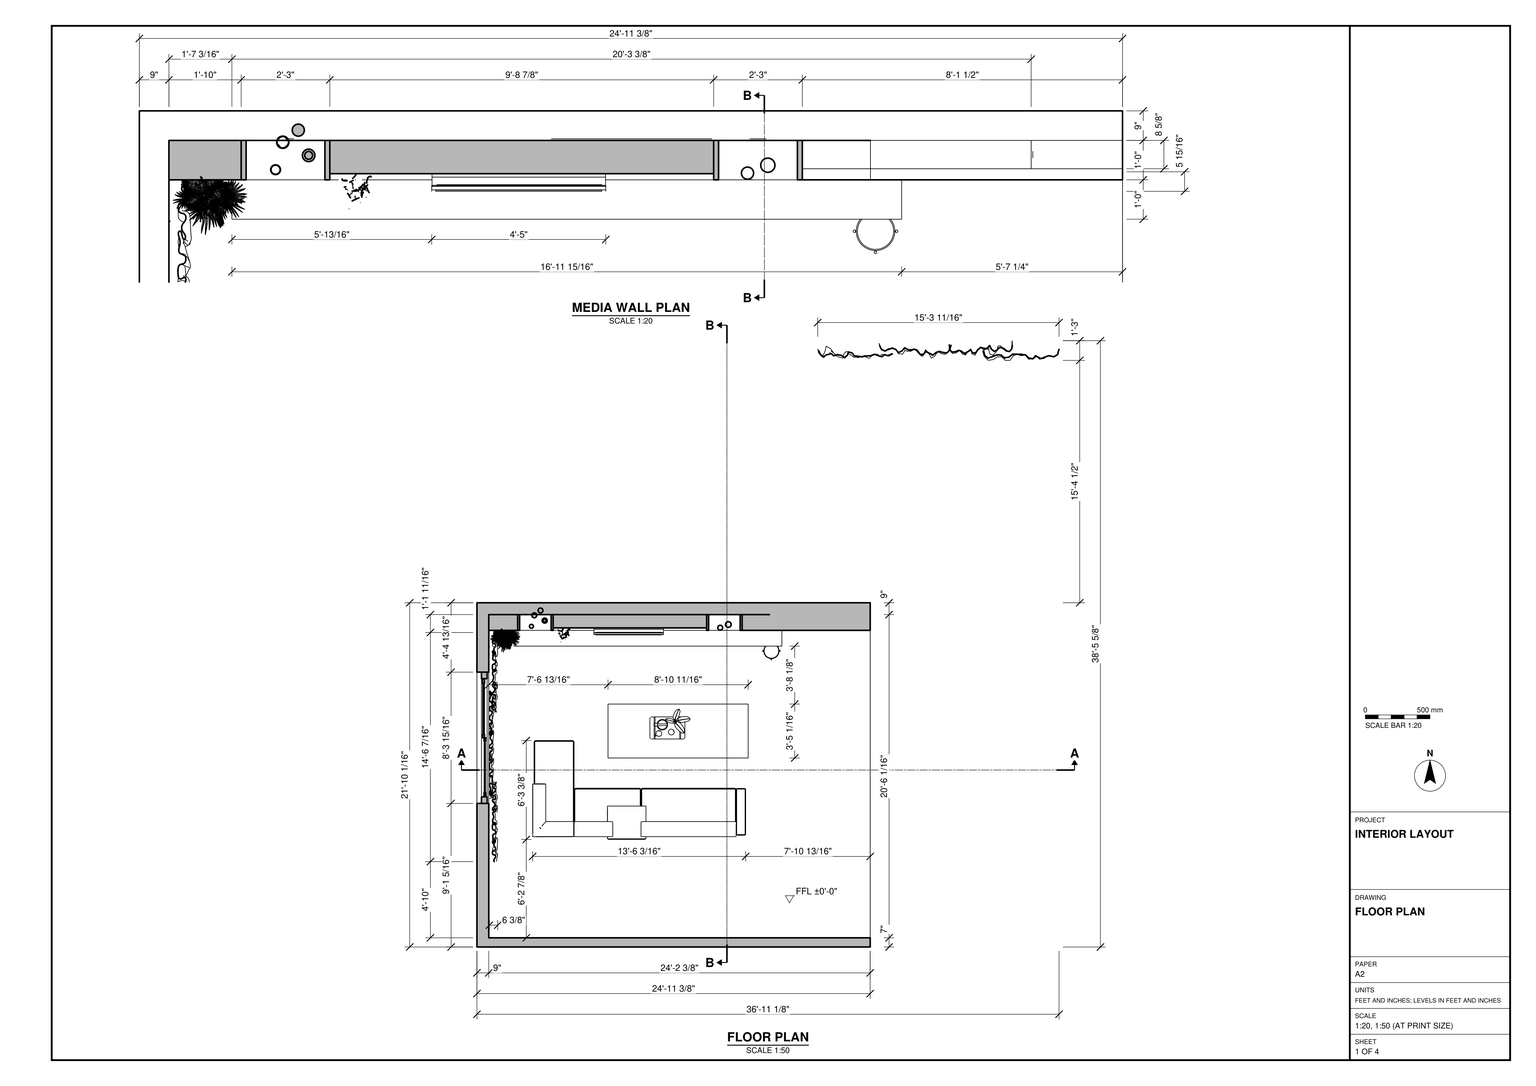
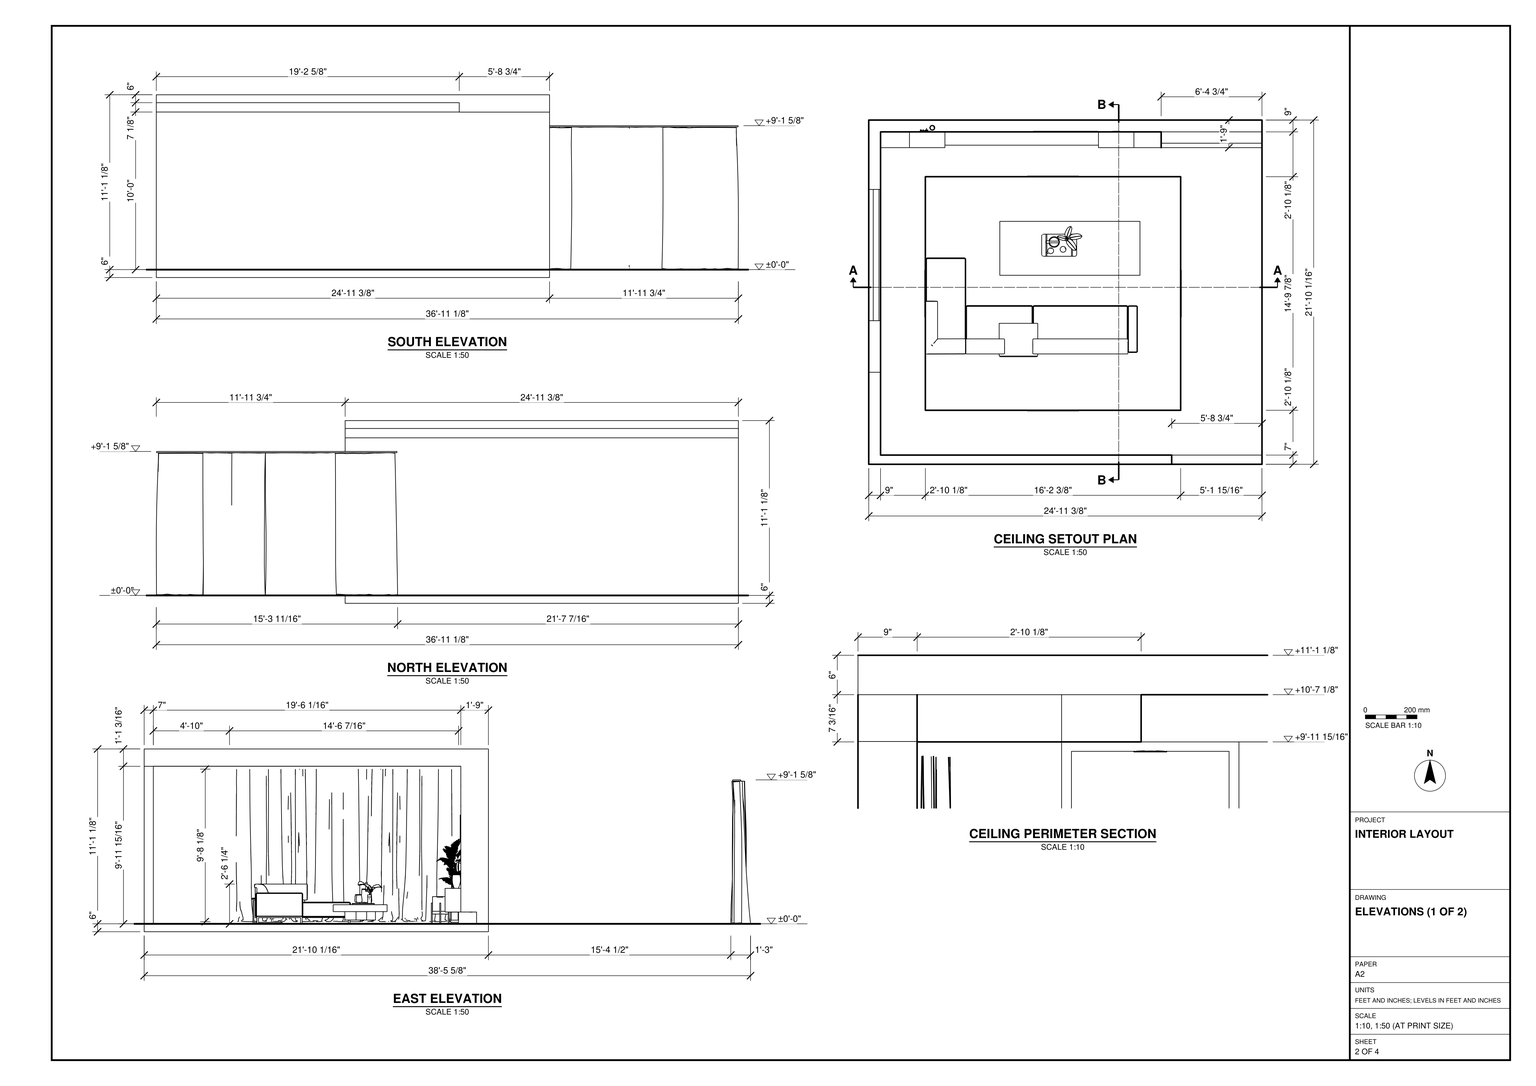
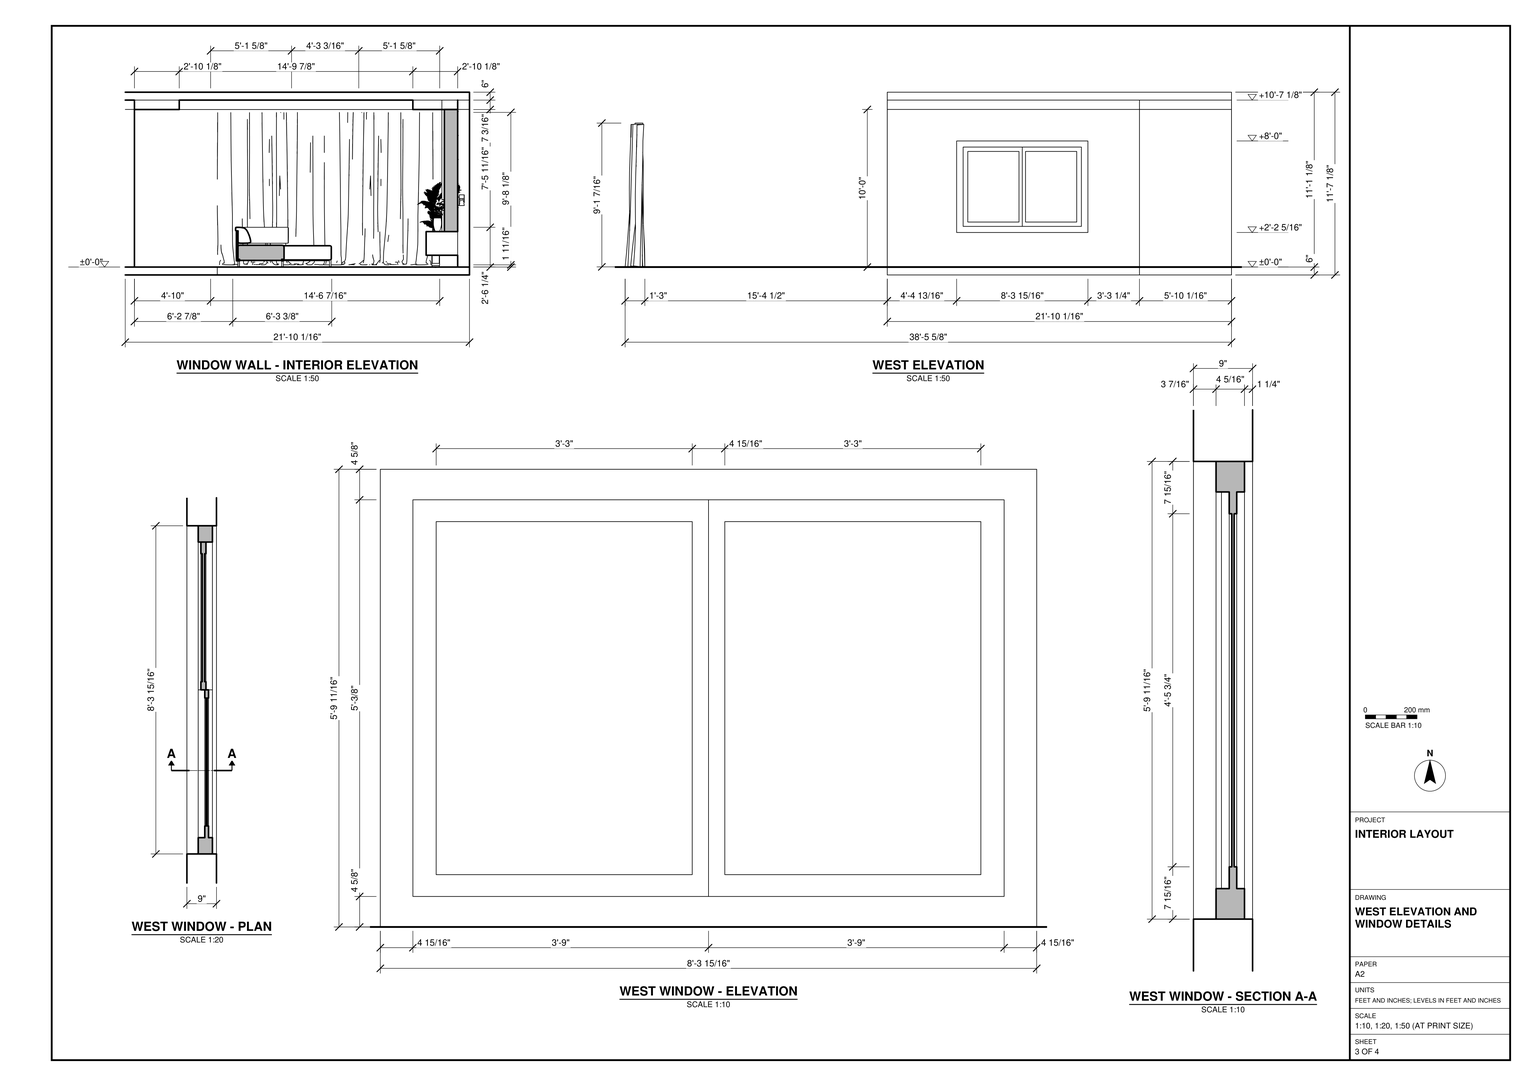
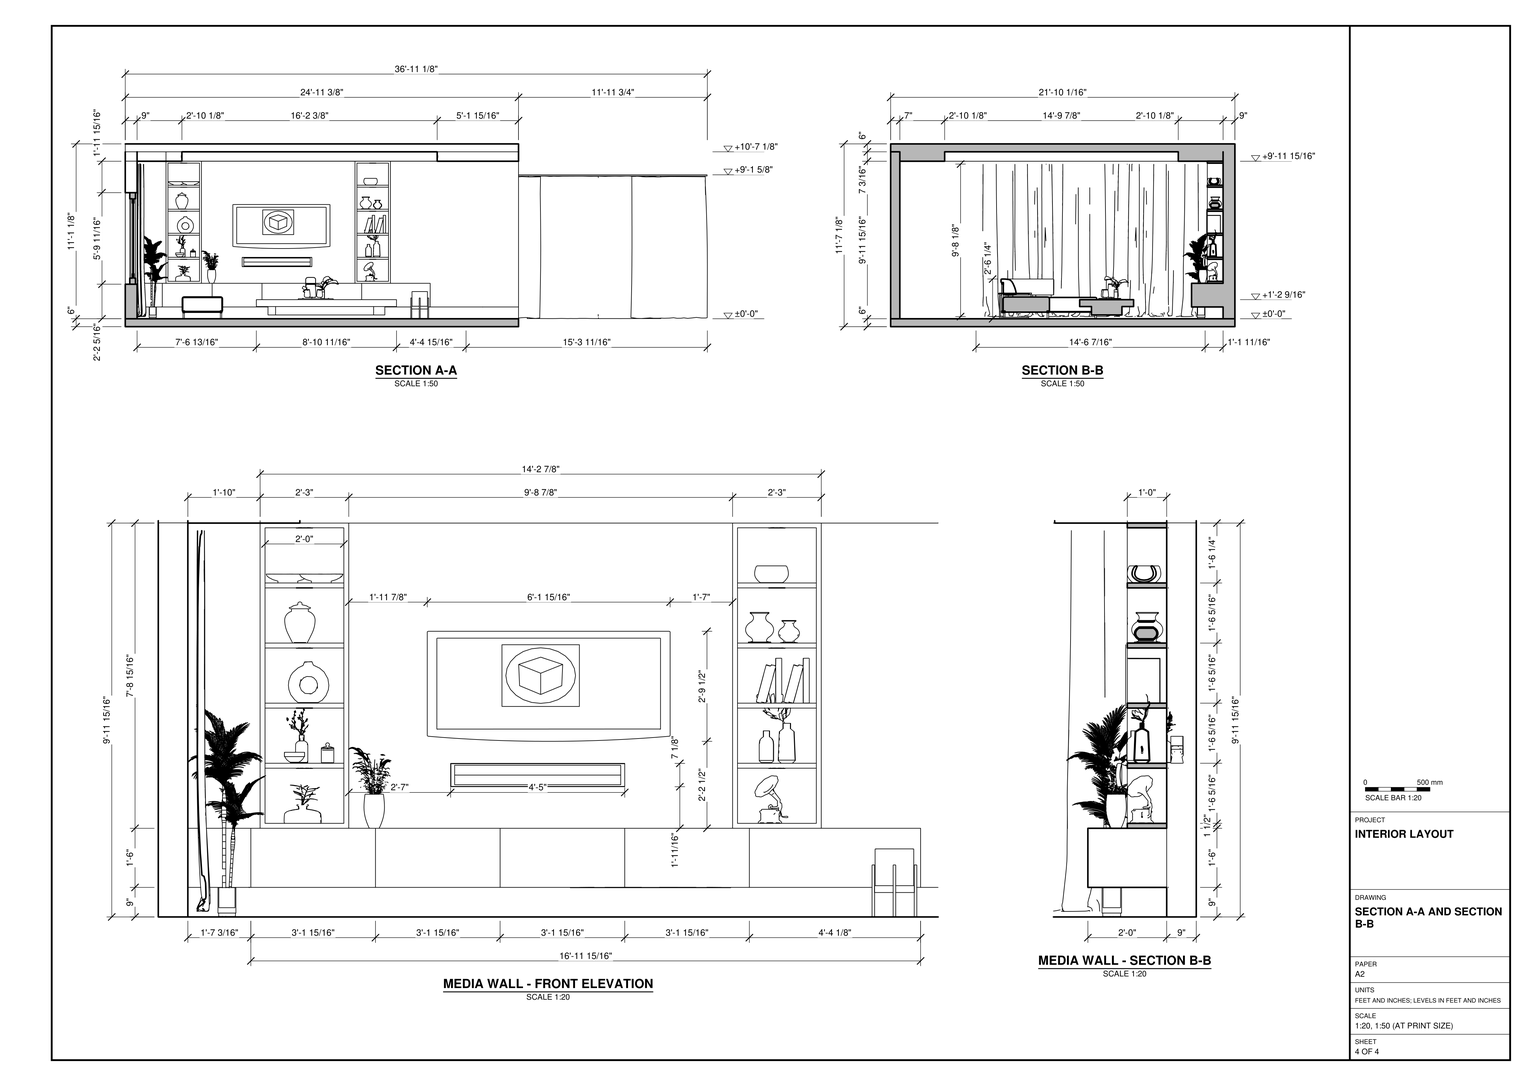
Build the living-room interior in SketchUp from task_files/diagram_01.pdf. Work in feet and inches, with the finished floor at ±0'-0". The complete model measures 36'-11 1/8" along X, 38'-5 5/8" along Y and 11'-7 1/8" along Z. These are not the room dimensions: the room shell measures 24'-11 3/8" across the media wall by 21'-10 1/16" along the window wall. Include the separate curtain run beyond the room where the floor plan and elevations show it.

Build the floor slab, the north and west walls at 9" thick and the south wall at 7" thick. Leave the east side open as drawn. Use the ceiling setout and perimeter section to form the lowered border around the recessed ceiling. Set the paired window into the west wall, with its frame, sill height and glazing taken from the window details, and place the interior curtains along that wall.

Use the enlarged media wall plan to set out the built-in bays, screen and projecting low unit on the north wall. Place the sectional sofa facing the screen, with its short return on the window side and the rectangular coffee table between the sofa and the media wall. Decor and loose items may be any suitable library components placed as shown. Keep shell elements and each furniture or joinery piece in separate groups or components, using components for repeated parts. Save one SketchUp model as output_files/living_room_with_its_media_wall_and_sectional_sofa.skp.

# SketchUp Ruby script. Lengths in inches.
U = 1.inch
M = Sketchup.active_model
def pt(a) = Geom::Point3d.new(a.map { |v| v * U })
def face(e, loops, mat)
  f = e.add_face(loops[0].map { |a| pt(a) })
  loops[1..].each { |l| e.add_face(l.map { |a| pt(a) }).erase! }
  f.material = f.back_material = mat if mat
  f
end
# faces: each face lists its corners as indices into pts; further lists are holes
def faces(e, pts, list, mat = nil) = list.each { |f| face(e, (f[0].is_a?(Array) ? f : [f]).map { |l| l.map { |i| pts[i] } }, mat) }
# xy, xz, yz: faces in a plane at the given z, y or x. An outline is a flat list of corners, or four numbers for a rectangle; further outlines are holes
def ring(l) = l.size == 4 ? [[l[0], l[1]], [l[2], l[1]], [l[2], l[3]], [l[0], l[3]]] : l.each_slice(2).to_a
def flat(e, list, mat, &to3) = list.each { |f| face(e, (f[0].is_a?(Array) ? f : [f]).map { |l| ring(l).map { |u, v| to3.(u, v) } }, mat) }
def xy(e, z, list, mat = nil) = flat(e, list, mat) { |x, y| [x, y, z] }
def xz(e, y, list, mat = nil) = flat(e, list, mat) { |x, z| [x, y, z] }
def yz(e, x, list, mat = nil) = flat(e, list, mat) { |y, z| [x, y, z] }
def lines(e, pts, list) = list.each { |a, b| e.add_line(pt(pts[a]), pt(pts[b])) }
# prism: a flat outline (further loops are holes) pulled along v
def prism(e, loops, v, mat = nil)
  f = face(e, loops, mat); d = Geom::Vector3d.new(v.map { |x| x * U })
  f.pushpull(f.normal.samedirection?(d) ? d.length : -d.length)
end
def box(e, o, s, mat = nil) = prism(e, [[o, [o[0] + s[0], o[1], o[2]], [o[0] + s[0], o[1] + s[1], o[2]], [o[0], o[1] + s[1], o[2]]]], [0, 0, s[2]], mat)
def at(x, y, z, deg = 0) = Geom::Transformation.translation(pt([x, y, z])) * Geom::Transformation.rotation(ORIGIN, Z_AXIS, deg.degrees)
def axes(o, x, y, z) = Geom::Transformation.new([*x, 0, *y, 0, *z, 0, *pt(o).to_a, 1])
def part(name) = M.definitions.add(name)
# library, detail: a bought-in or finely detailed component or shape, given as its bounding box
def library(name, o, s) = part(name).tap { |d| box(d.entities, o, s) }
def detail(e, o, s) = box(e.add_group.entities, o, s)
def put(e, d, t, mat = nil) = e.add_instance(d, t).tap { |i| i.material = mat if mat }
def group(e, t, mat = nil) = e.add_group.tap { |g| g.transformation = t; g.material = mat if mat }.entities
root = M.entities
M.materials.add("Generic").color = [37, 72, 93]
M.materials.add("Generic\#1").color = [217, 232, 252]
M.materials.add("Generic\#2").color = [244, 244, 245]
M.materials.add("Generic\#3").color = [100, 110, 121]
M.materials.add("[Translucent Glass Gray]").color = [128, 128, 128]
M.materials["[Translucent Glass Gray]"].alpha = 0.5
M.materials.add("[Translucent_Glass_Safety]").color = [204, 235, 244]
M.materials["[Translucent_Glass_Safety]"].alpha = 0.5
M.materials.add("[Translucent_Glass_Sky_Reflection]").color = [125, 138, 183]
M.materials["[Translucent_Glass_Sky_Reflection]"].alpha = 0.52
c1 = part("Sliding window")
xy(c1.entities,0,[[0,0,4.33,55.51]])
xy(c1.entities,2.76,[[0,2.76,2,27.76],[3.15,2.76,4.33,27.76],[0,27.76,0.82,52.76],[0.82,27.76,2.36,52.76],[2.36,27.76,4.33,52.76]])
xy(c1.entities,4.72,[[2,4.72,2.4,26.38],[2.76,4.72,3.15,26.38],[0.82,29.13,1.22,50.79],[1.97,29.13,2.36,50.79]])
xy(c1.entities,36.61,[[2,4.72,2.4,26.38],[2.76,4.72,3.15,26.38],[0.82,29.13,1.22,50.79],[1.97,29.13,2.36,50.79]])
xy(c1.entities,38.58,[[0,2.76,2,27.76],[3.15,2.76,4.33,27.76],[0,27.76,0.82,52.76],[0.82,27.76,2.36,52.76],[2.36,27.76,4.33,52.76]])
xy(c1.entities,41.34,[[0,0,4.33,55.51]])
xz(c1.entities,0,[[0,0,4.33,41.34]])
xz(c1.entities,2.76,[[0,2.76,2,38.58],[3.15,2.76,4.33,38.58]])
xz(c1.entities,4.72,[[2,4.72,2.4,36.61],[2.76,4.72,3.15,36.61]])
xz(c1.entities,26.38,[[2,4.72,2.4,36.61],[2.76,4.72,3.15,36.61]])
xz(c1.entities,27.76,[[0.82,2.76,2,38.58],[2,2.76,2.36,38.58],[2.36,2.76,3.15,38.58]])
xz(c1.entities,29.13,[[0.82,4.72,1.22,36.61],[1.97,4.72,2.36,36.61]])
xz(c1.entities,50.79,[[0.82,4.72,1.22,36.61],[1.97,4.72,2.36,36.61]])
xz(c1.entities,52.76,[[0,2.76,0.82,38.58],[0.82,2.76,2.36,38.58],[2.36,2.76,4.33,38.58]])
xz(c1.entities,55.51,[[0,0,4.33,41.34]])
yz(c1.entities,0,[[[0,0,55.51,41.34],[2.76,2.76,52.76,38.58]]])
yz(c1.entities,0.82,[[[27.76,2.76,52.76,38.58],[29.13,4.72,50.79,36.61]]])
yz(c1.entities,1.22,[[29.13,4.72,50.79,36.61]],"[Translucent_Glass_Sky_Reflection]")
yz(c1.entities,1.97,[[29.13,4.72,50.79,36.61]],"[Translucent_Glass_Sky_Reflection]")
yz(c1.entities,2,[[[2.76,2.76,27.76,38.58],[4.72,4.72,26.38,36.61]]])
yz(c1.entities,2.36,[[[27.76,2.76,52.76,38.58],[29.13,4.72,50.79,36.61]]])
yz(c1.entities,2.4,[[4.72,4.72,26.38,36.61]],"[Translucent_Glass_Safety]")
yz(c1.entities,2.76,[[4.72,4.72,26.38,36.61]],"[Translucent_Glass_Safety]")
yz(c1.entities,3.15,[[[2.76,2.76,27.76,38.58],[4.72,4.72,26.38,36.61]]])
yz(c1.entities,4.33,[[[0,0,55.51,41.34],[2.76,2.76,52.76,38.58]]])
c2 = library("sofa 2",[0,0,0],[184.3,73.16,30.26])
c3 = library("Bowl\#1",[-1.49,-1.48,0],[2.98,2.96,1.18])
c4 = library("stone+Jar+4",[7.875,-15.36,0],[26.34,31.07,40.68])
c5 = library("Gramophone 194 010",[-11.96,-11.51,-0.03],[26.29,20.83,37.93])
c6 = library("Books 297 001 006",[-2.01,-2.6,-0.02],[4.03,5.2,7.13])
c7 = library("Vase 274 006 003",[-5.27,-1.49,-0.03],[10.54,2.98,10.64])
c8 = library("Plant1",[-0.09,-1.87,0],[3.22,5.78,8.62])
c9 = library("Untitled (9)",[-0.59,0,0],[15.67,17.07,16.5])
c10 = library("Plant",[-27.84,-31.84,-1.26],[68.28,70.82,154.38])
c11 = library("PLATE - KITCHEN",[0,-1.1875,0],[35.61,27.27,18.32])
c12 = library("Lidded jar",[0,0,0],[13.42,13.42,18.18])
c13 = library("Raised planter",[1.65,0,0],[13.63,13.63,20.73])
c14 = library("Group3\#1",[-238.15,54.18,0],[46.4,43.96,56.68])
c15 = library("Untitled\#1",[82.71,28.87,-11.8125],[39.77,1.97,25.2])
c16 = library("Wisdom Sage Series P38m ( On Wall )",[6.24,4.69,38.8125],[7.11,5.95,34.2])
c17 = library("Curtains 001",[-91.88,-6.87,0.16],[183.71,15.03,109.46])
c18 = library("Group\#2",[0,0,0],[6.18,105.6875,105.34])
c19 = library("Group\#27",[-0.5,-0.5,0],[117.875,2.875,93])
c20 = library("Group\#28",[-0.5,-0.5,-0.1],[25,3.75,0.2])
c21 = library("Group\#29",[-0.5,-0.5,-0.1],[25,4.125,0.2])
c22 = library("Group\#30",[-0.5,-0.5,-0.1],[25,4.0625,0.2])
c23 = library("Group\#31",[-0.5,-0.5,-0.1],[25,3.875,0.2])
c24 = library("Group\#32",[-0.5,-0.5,-0.1],[25,3.5625,0.2])
c25 = library("Group\#33",[-0.5,-0.5,-0.1],[25,4,0.2])
c26 = library("Group\#34",[-0.5,-0.5,-0.1],[25,3.87,0.2])
c27 = library("Group\#35",[-0.5,-0.5,-0.1],[25,3.25,0.2])
c28 = library("Group\#36",[-0.5,-0.5,-0.1],[25,3.8125,0.2])
c29 = library("Group\#37",[-0.5,-0.5,-0.1],[25,4.25,0.2])
c30 = library("Group\#38",[-0.5,-0.5,0],[195.35,178.85,7.1875])
c31 = library("Mesh Light\#12",[-0.5,-0.5,-0.1],[1,1,0.2])
xy(root,-6,[[0,0,230.625,70.0625],[230.625,0,230.625,70.0625,0,70.0625,0,262.0625,299.375,262.0625,299.375,0]])
xy(root,0,[[0,0,299.375,0,299.375,7,9,7,9,70.0625,0,70.0625],[0,70.0625,9,70.0625,9,253.0625,299.375,253.0625,299.375,262.0625,0,262.0625]])
xy(root,0,[[9,7,299.375,253.0625]],"Generic\#2")
xy(root,9,[[28.18,229.0625,28.18,244.4375,299.375,244.4375,299.375,241.0625,232.125,241.0625,232.125,229.0625],[271.5625,244.4375,299.375,253.0625]])
xy(root,26.3125,[[0,109.3125,9,209.25]])
xy(root,27,[[9,241.0625,28.18,253.0625],[28.18,241.0625,31,253.0625],[31,241.0625,58,253.0625],[174.875,241.0625,201.875,253.0625],[58,242.9375,174.875,253.0625]])
xy(root,27,[[28.18,229.0625,232.125,241.0625]],"Generic")
xy(root,28.5,[[32.5,241.0625,56.5,253.0625],[176.375,241.0625,200.375,253.0625]],"Generic\#3")
xy(root,45.3,[[32.5,241.0625,56.5,249.8125],[176.375,241.0625,200.375,250.3125]])
xy(root,46.8,[[32.5,241.0625,56.5,253.0625],[176.375,241.0625,200.375,253.0625]],"Generic\#3")
xy(root,63.6,[[32.5,241.0625,56.5,250.25],[176.375,241.0625,200.375,249.9375]])
xy(root,65.1,[[32.5,241.0625,56.5,253.0625],[176.375,241.0625,200.375,253.0625]],"Generic\#3")
xy(root,81.9,[[32.5,241.0625,56.5,250.8125],[176.375,241.0625,200.375,250]])
xy(root,83.4,[[32.5,241.0625,56.5,253.0625],[176.375,241.0625,200.375,253.0625]],"Generic\#3")
xy(root,96,[[0,109.3125,9,209.25]])
xy(root,100.2,[[32.5,241.0625,56.5,250.2]])
xy(root,100.2,[[176.375,241.0625,200.375,250.5]],"Generic\#3")
xy(root,101.7,[[32.5,241.0625,56.5,253.0625],[176.375,241.0625,200.375,253.0625]],"Generic\#3")
xy(root,118.5,[[32.5,241.0625,56.5,250.0625]])
xy(root,118.5,[[176.375,241.0625,200.375,250.1875]],"Generic\#3")
xy(root,119.9375,[[230.625,0,299.375,7],[[9,7,299.375,7,299.375,241.0625,222.625,241.0625,222.625,253.0625,9,253.0625],[43.11,41.11,237.45,218.95]]])
xy(root,120,[[9,241.0625,31,253.0625],[31,241.0625,58,253.0625],[174.875,241.0625,201.875,253.0625],[201.875,241.0625,222.625,253.0625],[58,242.9375,174.875,253.0625]])
xy(root,127.125,[[0,0,230.625,0,230.625,7,9,7,9,70.0625,0,70.0625]])
xy(root,127.125,[[43.11,41.11,237.45,218.95]],"Generic\#2")
xy(root,133.125,[[0,0,299.375,262.0625]])
xz(root,0,[[0,-6,299.375,0],[0,0,299.375,0,299.375,119.9375,230.625,119.9375,230.625,120,0,120],[230.625,119.9375,230.625,127.125,0,127.125,0,133.125,299.375,133.125,299.375,119.9375],[0,120,230.625,127.125]])
xz(root,7,[[9,119.9375,230.625,120],[9,120,230.625,127.125]])
xz(root,7,[[9,0,299.375,119.9375]],"Generic\#1")
xz(root,109.3125,[[0,26.3125,9,96]])
xz(root,209.25,[[0,26.3125,9,96]])
xz(root,229.0625,[[28.18,9,66.13,27],[66.13,9,104.08,27],[104.08,9,142.04,27],[142.04,9,179.99,27],[179.99,9,232.125,27]],"Generic")
xz(root,241.0625,[[222.625,119.9375,299.375,120]])
xz(root,241.0625,[[232.125,9,299.375,9,299.375,119.9375,222.625,119.9375,222.625,120,201.875,120,201.875,27,232.125,27],[9,27,31,120]],"Generic\#1")
xz(root,241.0625,[[[31,27,58,120],[32.5,28.5,56.5,118.5]],[[174.875,27,201.875,120],[176.375,28.5,200.375,118.5]],[32.5,45.3,56.5,46.8],[176.375,45.3,200.375,46.8],[32.5,63.6,56.5,65.1],
  [176.375,63.6,200.375,65.1],[32.5,81.9,56.5,83.4],[176.375,81.9,200.375,83.4],[32.5,100.2,56.5,101.7],[176.375,100.2,200.375,101.7]],"Generic\#2")
xz(root,242.9375,[[58,27,174.875,120]],"Generic\#1")
xz(root,253.0625,[[9,9,28.18,27],[9,27,31,119.9375],[[31,27,58,119.9375],[32.5,65.1,56.5,81.9],[32.5,28.5,56.5,45.3],[32.5,46.8,56.5,63.6],[32.5,83.4,56.5,100.2],[32.5,101.7,56.5,118.5]],[58,27,174.875,119.9375],[[174.875,27,201.875,119.9375],[176.375,65.1,200.375,81.9],[176.375,28.5,200.375,45.3],[176.375,46.8,200.375,63.6],[176.375,83.4,200.375,100.2],[176.375,101.7,200.375,118.5]],
  [201.875,27,222.625,119.9375],[9,119.9375,31,120],[31,119.9375,58,120],[58,119.9375,174.875,120],[174.875,119.9375,201.875,120],
  [201.875,119.9375,222.625,120],[9,120,31,127.125],[31,120,58,127.125],[58,120,174.875,127.125],[174.875,120,201.875,127.125],
  [201.875,120,222.625,127.125]])
xz(root,253.0625,[[9,0,299.375,9]],"Generic\#2")
xz(root,253.0625,[[32.5,28.5,56.5,45.3],[176.375,28.5,200.375,45.3],[32.5,46.8,56.5,63.6],[176.375,46.8,200.375,63.6],[32.5,65.1,56.5,81.9],
  [176.375,65.1,200.375,81.9],[32.5,83.4,56.5,100.2],[176.375,83.4,200.375,100.2],[32.5,101.7,56.5,118.5],[176.375,101.7,200.375,118.5]],"Generic\#3")
xz(root,262.0625,[[0,-6,299.375,0],[0,0,299.375,120],[0,120,299.375,127.125],[0,127.125,299.375,133.125]])
yz(root,0,[[0,-6,70.0625,0],[70.0625,-6,262.0625,0],[0,0,70.0625,120],[[70.0625,0,262.0625,120],[109.3125,26.3125,209.25,96]],[0,120,70.0625,127.125],
  [70.0625,120,262.0625,127.125]])
yz(root,9,[[241.0625,27,253.0625,119.9375],[7,119.9375,70.0625,120],[70.0625,119.9375,241.0625,120],[241.0625,119.9375,253.0625,120],[7,120,70.0625,127.125],
  [70.0625,120,241.0625,127.125],[241.0625,120,253.0625,127.125]])
yz(root,9,[[[7,0,253.0625,0,253.0625,27,241.0625,27,241.0625,119.9375,7,119.9375],[109.3125,26.3125,209.25,96]]],"Generic\#1")
yz(root,28.18,[[229.0625,9,253.0625,27]],"Generic")
yz(root,31,[[241.0625,27,253.0625,120]])
yz(root,32.5,[[241.0625,28.5,253.0625,45.3],[241.0625,46.8,253.0625,63.6],[241.0625,65.1,253.0625,81.9],[241.0625,83.4,253.0625,100.2],[241.0625,101.7,253.0625,118.5]],"Generic\#3")
yz(root,56.5,[[241.0625,28.5,253.0625,45.3],[241.0625,46.8,253.0625,63.6],[241.0625,65.1,253.0625,81.9],[241.0625,83.4,253.0625,100.2],[241.0625,101.7,253.0625,118.5]],"Generic\#3")
yz(root,58,[[242.9375,27,253.0625,120]])
yz(root,174.875,[[242.9375,27,253.0625,118.5],[242.9375,118.5,253.0625,120]])
yz(root,176.375,[[241.0625,28.5,253.0625,45.3],[241.0625,46.8,253.0625,63.6],[241.0625,65.1,253.0625,81.9],[241.0625,83.4,253.0625,100.2],[241.0625,101.7,253.0625,118.5]],"Generic\#3")
yz(root,200.375,[[241.0625,28.5,253.0625,45.3],[241.0625,46.8,253.0625,63.6],[241.0625,65.1,253.0625,81.9],[241.0625,83.4,253.0625,100.2],[241.0625,101.7,253.0625,118.5]],"Generic\#3")
yz(root,201.875,[[241.0625,27,253.0625,118.5],[241.0625,118.5,253.0625,120]])
yz(root,222.625,[[241.0625,119.9375,253.0625,120],[241.0625,120,253.0625,127.125]])
yz(root,230.625,[[0,119.9375,7,120],[0,120,7,127.125]])
yz(root,232.125,[[229.0625,9,241.0625,27]],"Generic")
yz(root,237.45,[[41.11,119.9375,218.95,127.125]])
yz(root,299.375,[[0,-6,262.0625,0],[0,0,7,119.9375],[253.0625,0,253.0625,9,241.0625,9,241.0625,119.9375,0,119.9375,0,133.125,262.0625,133.125,262.0625,0]])
p = [[230.625,70.0625,0],[230.625,70.0625,-6],[222.625,253.0625,27],[222.625,241.0625,27],[222.625,241.0625,127.125],[299.375,241.0625,127.125]]
lines(root,p,[[0,1],[2,3],[4,5]])
detail(root,[32.86,241.26,101.34],[23.36,11.89,3.06])
detail(root,[188.74,242.89,46.8],[5.26,5.25,12.17])
detail(root,[189.55,245.32,49.8],[2.52,0.77,9.87])
detail(root,[182.15,242.24,59.65],[10.35,5.91,9.04])
detail(root,[182.98,240.89,47.02],[4.41,4.41,9.65])
put(root,c1,axes([3.4375,109.3125,26.3125],[1,0,0],[0,1.80029,0],[0,0,1.68577]))
put(root,c2,axes([204.57,157.21,0],[-0.88,0,0],[0,-1.03,0],[0,0,1]))
put(root,c3,axes([186.72,246.17,101.7],[3.458,0,0],[0,3.458,0],[0,0,4.42624]))
put(root,c4,axes([176.27,247.09,83.55],[0.32433,0,0],[0,0.3051,0],[0,0,0.226]))
put(root,c4,axes([186.92,246.79,83.4],[0.24325,0,0],[0,0.22883,0],[0,0,0.1695]))
put(root,c5,axes([186.25,245.46,28.51],[0.3822,0,0],[0,0.3822,0],[0,0,0.3822]))
put(root,c6,axes([194.34,246.07,65.14],[1.9215,0,0],[0,1.9215,0],[0,0,1.9215]))
put(root,c6,axes([185.96,246.07,65.14],[1.9215,0,0],[0,1.9215,0],[0,0,1.9215]),"[Translucent Glass Gray]")
put(root,c7,axes([45.77,244.92,65.33],[1.17,0,0],[0,-1.26511,0],[0,0,1.17]))
put(root,c8,axes([38.3125,245.13,28.5],[3.7184,0,0],[0,1.66,0],[0,0,1.66]))
put(root,c9,at(38.38,241.0625,46.8))
put(root,c10,axes([17.48,233.04,0.14],[0.43,0,0],[0,0.43,0],[0,0,0.43]))
put(root,c11,at(131.65,158.35,14.5625))
put(root,c12,axes([38.49,241.0625,83.4],[0.69,0,0],[0,0.69,0],[0,0,0.69]),"[Translucent Glass Gray]")
put(root,c13,at(215.69,218.59,0))
put(root,c14,axes([163.73,203.92,26.86],[0.4608,0,0],[0,0.4608,0],[0,0,0.4608]))
put(root,c15,axes([-71.95,212.57,69.19],[1.86,0,0],[0,1,0],[0,0,1.33]))
put(root,c16,axes([202.19,232.87,33.42],[0,0,1],[0,1,0],[-1.55,0,0]))
put(root,c17,at(351.29,453.45,0))
put(root,c18,axes([9.45,64.98,1.68],[1.03,0,0],[0,1.65037,0],[0,0,1.1021]))
g1 = group(root,at(99.78,143.89,2.91))
detail(g1,[0,0,0],[106.7,41.05,11.65])
put(root,c19,at(58,241.0625,27))
put(root,c20,at(176.375,250.3125,45.3))
put(root,c21,at(176.375,249.9375,63.6))
put(root,c22,at(176.375,250,81.9))
put(root,c23,at(176.375,250.1875,118.5))
put(root,c24,at(176.375,250.5,100.2))
put(root,c25,at(32.5,250.0625,118.5))
put(root,c26,at(32.5,250.2,100.2))
put(root,c27,at(32.5,250.8125,81.9))
put(root,c28,at(32.5,250.25,63.6))
put(root,c29,at(32.5,249.8125,45.3))
put(root,c30,at(43.11,41.11,119.9375))
g2 = group(root,at(28.18,244.4375,9))
xy(g2,0,[[0,0,243.38,8.625]])
put(g2,c31,axes([121.69,4.3125,0],[244.38025,0,0],[0,9.625,0],[0,0,1]))
